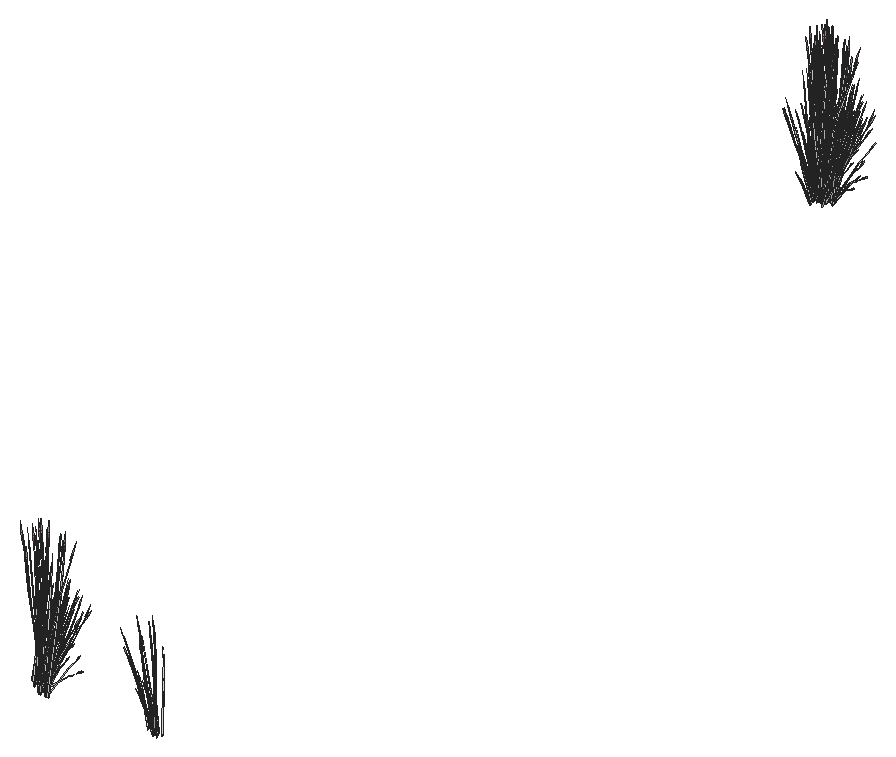
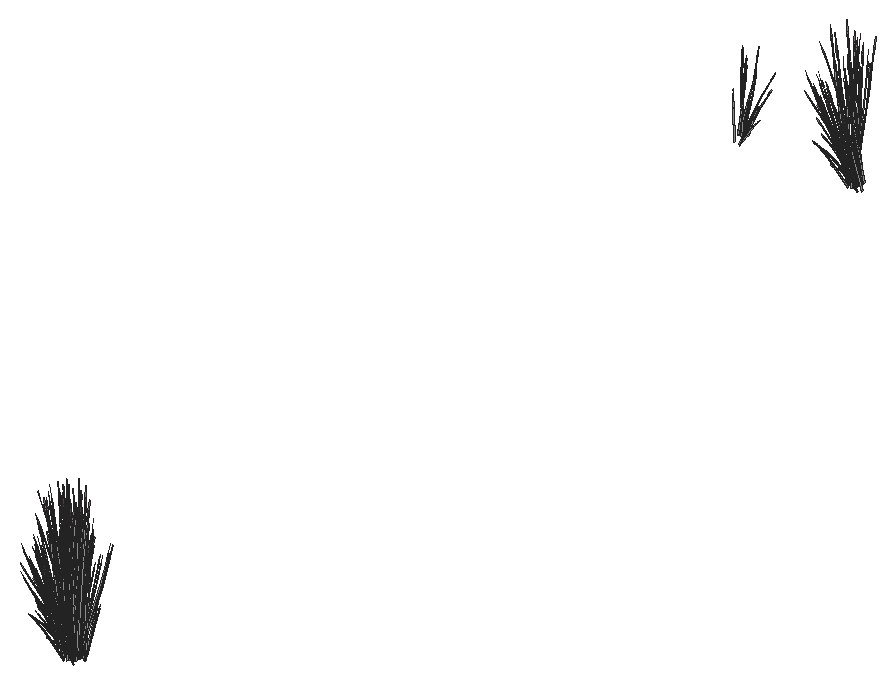
# SketchUp Ruby script. Lengths in inches.
U = 1.inch
M = Sketchup.active_model
def pt(a) = Geom::Point3d.new(a.map { |v| v * U })
def face(e, loops, mat)
  f = e.add_face(loops[0].map { |a| pt(a) })
  loops[1..].each { |l| e.add_face(l.map { |a| pt(a) }).erase! }
  f.material = f.back_material = mat if mat
  f
end
# faces: each face lists its corners as indices into pts; further lists are holes
def faces(e, pts, list, mat = nil) = list.each { |f| face(e, (f[0].is_a?(Array) ? f : [f]).map { |l| l.map { |i| pts[i] } }, mat) }
# xy, xz, yz: faces in a plane at the given z, y or x. An outline is a flat list of corners, or four numbers for a rectangle; further outlines are holes
def ring(l) = l.size == 4 ? [[l[0], l[1]], [l[2], l[1]], [l[2], l[3]], [l[0], l[3]]] : l.each_slice(2).to_a
def flat(e, list, mat, &to3) = list.each { |f| face(e, (f[0].is_a?(Array) ? f : [f]).map { |l| ring(l).map { |u, v| to3.(u, v) } }, mat) }
def xy(e, z, list, mat = nil) = flat(e, list, mat) { |x, y| [x, y, z] }
def xz(e, y, list, mat = nil) = flat(e, list, mat) { |x, z| [x, y, z] }
def yz(e, x, list, mat = nil) = flat(e, list, mat) { |y, z| [x, y, z] }
def lines(e, pts, list) = list.each { |a, b| e.add_line(pt(pts[a]), pt(pts[b])) }
# prism: a flat outline (further loops are holes) pulled along v
def prism(e, loops, v, mat = nil)
  f = face(e, loops, mat); d = Geom::Vector3d.new(v.map { |x| x * U })
  f.pushpull(f.normal.samedirection?(d) ? d.length : -d.length)
end
def box(e, o, s, mat = nil) = prism(e, [[o, [o[0] + s[0], o[1], o[2]], [o[0] + s[0], o[1] + s[1], o[2]], [o[0], o[1] + s[1], o[2]]]], [0, 0, s[2]], mat)
def at(x, y, z, deg = 0) = Geom::Transformation.translation(pt([x, y, z])) * Geom::Transformation.rotation(ORIGIN, Z_AXIS, deg.degrees)
def axes(o, x, y, z) = Geom::Transformation.new([*x, 0, *y, 0, *z, 0, *pt(o).to_a, 1])
def part(name) = M.definitions.add(name)
# library, detail: a bought-in or finely detailed component or shape, given as its bounding box
def library(name, o, s) = part(name).tap { |d| box(d.entities, o, s) }
def detail(e, o, s) = box(e.add_group.entities, o, s)
def put(e, d, t, mat = nil) = e.add_instance(d, t).tap { |i| i.material = mat if mat }
def group(e, t, mat = nil) = e.add_group.tap { |g| g.transformation = t; g.material = mat if mat }.entities
root = M.entities
M.materials.add("LightPink_Translucent").color = [144, 107, 117]
M.materials["LightPink_Translucent"].alpha = 0.75
c1 = part("blade")
p = [[2.15,0.21,22],[0,0.17,0],[0.09,0.45,0],[2.18,0.31,22],[2.29,0.31,22],[0.38,0.45,0],
  [2.48,0.24,33],[2.49,0.24,33],[2.48,0.22,33]]
faces(c1.entities,p,[[0,1,2,3],[4,5,2,3],[6,3,4,7],[8,0,3,6]])
c2 = part("seeds")
p = [[0.3,-0.1,1.38],[-0.01,-0.03,1.59],[-0.01,-0.03,0.03],[0.14,-0.07,-0.07],[0.29,-0.03,3],[0.15,0.01,3.11]]
faces(c2.entities,p,[[0,1,2,3],[1,0,4,5]],"LightPink_Translucent")
c3 = part("blade with seeds")
put(c3.entities,c1,at(0,0,0))
put(c3.entities,c2,axes([2.4,0.25,30.99],[1.5799,-0.05474,1.17369],[-0.12525,1.92788,0.29478],[-0.07173,-0.02425,1.56792]))
put(root,c3,axes([698.92,479.98,4.52],[-0.44971,0.15222,-0.0608],[-0.221,-0.27017,-0.33747],[-0.05933,-0.11385,0.51278]))
put(root,c3,axes([698.54,480,4.34],[-0.45175,-0.08196,-0.25549],[0.15485,-0.28101,-0.1979],[-0.04142,-0.11314,0.48886]))
put(root,c3,axes([697.7,482.08,3.9375],[-0.01125,-0.12549,0.85688],[0.48751,0.08325,0.06928],[-0.03015,0.17883,0.36631]))
put(root,c3,axes([696.8,481.01,3.01],[0.32079,-0.20399,-0.15489],[0.32079,0.20399,0.15489],[0,-0.06571,0.69487]))
put(root,c3,axes([699.8,281.16,1.01],[-0.4301,0.16348,-0.24825],[-0.25708,-0.29314,0],[-0.09796,0.03723,0.78752]))
put(root,c3,axes([698.24,479.69,3.0625],[-0.31757,0.18757,-0.01946],[-0.29098,-0.20543,-0.08825],[-0.02049,-0.05821,0.29107]))
put(root,c3,axes([699.83,281.07,1.1],[-0.28374,-0.32877,-0.02571],[0.4807,-0.18271,0.25804],[-0.11845,0.0313,0.81815]))
put(root,c3,axes([698.12,481.54,3.18],[0.58084,0.06889,0.22877],[-0.11821,0.38906,0.08977],[-0.08488,-0.03757,0.79428]))
put(root,c3,axes([698.01,280.92,2.5],[0.32898,0.21969,-0.2836],[-0.34753,0.1924,-0.21967],[-0.05006,0.11162,0.54264]))
put(root,c3,axes([699.7,281.03,1.01],[-0.42874,-0.0809,-0.15489],[0.10795,-0.28489,0.15489],[-0.08643,0.03285,0.69487]))
put(root,c3,axes([697.97,481.47,3.36],[-0.22297,0.29461,0.2237],[-0.4633,-0.14179,-0.10766],[0,-0.06791,0.71822]))
put(root,c3,axes([698.7,480.05,4.49],[-0.21934,-0.26585,-0.35523],[0.45151,-0.14816,0.04287],[-0.05129,-0.12845,0.5025]))
put(root,c3,axes([697.86,280.76,2.53],[0.31095,-0.17214,0.17707],[0.29435,0.19656,-0.2286],[-0.04479,0.09987,0.4374]))
put(root,c3,axes([699.95,279.81,1.42],[-0.01255,-0.30784,0.70636],[0.56816,0.0798,0.29908],[-0.13438,0.16845,0.66675]))
put(root,c3,axes([697.8,482.16,3.24],[0.49383,-0.08678,0.08821],[0.12194,0.32295,0.17543],[-0.04404,-0.04705,0.80203]))
put(root,c3,axes([697.66,280.81,2.7],[0.50507,0.0162,-0.06749],[-0.01381,0.30672,-0.3746],[-0.03508,0.11813,0.56919]))
put(root,c3,axes([697.65,281.25,1.41],[0.41748,-0.0579,0.03254],[0.09598,0.23326,-0.43152],[-0.02647,0.11808,0.3868]))
put(root,c3,axes([699.625,280.2,1.33],[0.05355,0.37308,-0.14548],[-0.55775,0.02256,-0.25001],[-0.09822,0.04969,0.79854]))
put(root,c3,axes([698.44,482.21,3.1],[-0.4633,-0.14679,0],[0.22297,-0.30501,0],[0,0,0.81353]))
put(root,c3,axes([698.79,480.09,4.53],[-0.13855,0.25143,0.17707],[-0.4042,-0.07334,-0.2286],[-0.03706,-0.10123,0.4374]))
put(root,c3,axes([699.51,482.58,3.1875],[0.28732,0.32763,0],[-0.4807,0.18271,-0.25804],[-0.10948,0.04161,0.81856]))
put(root,c3,axes([698.38,280.61,1.9375],[-0.01125,-0.12549,0.85688],[0.48751,0.08325,0.06928],[-0.03015,0.17883,0.36631]))
put(root,c3,axes([698.05,482.72,4.53],[-0.45283,-0.08548,0.26641],[0.15485,-0.28101,0.21967],[0.02721,0.11051,0.55128]))
put(root,c3,axes([697.93,482.74,4.37],[-0.33863,0.11112,0.03215],[-0.16575,-0.20263,0.2531],[0.0327,0.08932,0.38595]))
put(root,c3,axes([699.27,482.18,3.24],[0.13276,-0.32494,0.08821],[0.4858,0.09195,0.17543],[-0.08392,0.00158,0.80203]))
put(root,c3,axes([699.05,481.75,3.31],[0.33952,0.19644,0.0724],[-0.2832,0.22163,-0.20674],[-0.07883,0.02996,0.63372]))
put(root,c3,axes([698.93,481.51,3.15],[-0.42746,-0.28142,-0.03066],[0.42772,-0.28159,0],[-0.01493,-0.00983,0.87786]))
put(root,c3,axes([699.04,481.6,3.36],[0.49904,-0.02018,0.2237],[0.04513,0.33504,-0.10766],[-0.08934,0.03396,0.71822]))
put(root,c3,axes([699.16,482.375,3.17],[0.57533,0.10627,0.15378],[-0.14394,0.37986,-0.18246],[-0.09522,0.04754,0.82443]))
put(root,c3,axes([698.32,479.46,2.75],[-0.07708,0.01178,0.88171],[-0.42627,-0.1326,-0.1347],[0.00715,-0.1106,0.15018]))
put(root,c3,axes([699.41,482.35,3.24],[0.4301,-0.16348,0.24825],[0.25708,0.29314,0],[-0.09796,0.03723,0.78752]))
put(root,c3,axes([698.74,479.82,4.26],[0.13855,-0.25143,-0.17707],[0.4042,0.07334,0.2286],[-0.03706,-0.10123,0.4374]))
put(root,c3,axes([698.07,481.18,3.18],[0.1998,0.3656,0.22877],[-0.5709,0.12713,0.08977],[0.00698,-0.06718,0.79428]))
put(root,c3,axes([697.98,481.14,3.11],[0.22297,-0.29461,-0.2237],[0.4633,0.14179,0.10766],[0,-0.06791,0.71822]))
put(root,c3,axes([698.55,482.09,3.1],[-0.14994,-0.28188,0],[0.42817,-0.09871,0],[0,0,0.77185]))
put(root,c3,axes([698,482.68,2.75],[0.07437,-0.01779,0.88171],[0.44738,0.09793,-0.1347],[0.01308,0.11037,0.15018]))
put(root,c3,axes([698.1,482.78,4.26],[-0.13855,0.25143,-0.17707],[-0.4042,-0.07334,0.2286],[0.03706,0.10123,0.4374]))
put(root,c3,axes([700.19,281.11,1.1875],[0.28732,0.32763,0],[-0.4807,0.18271,-0.25804],[-0.10948,0.04161,0.81856]))
put(root,c3,axes([698.73,281.25,2.53],[-0.45283,-0.08548,0.26641],[0.15485,-0.28101,0.21967],[0.02721,0.11051,0.55128]))
put(root,c3,axes([698.61,281.27,2.37],[-0.33863,0.11112,0.03215],[-0.16575,-0.20263,0.2531],[0.0327,0.08932,0.38595]))
put(root,c3,axes([699.73,280.27,1.31],[0.33952,0.19644,0.0724],[-0.2832,0.22163,-0.20674],[-0.07883,0.02996,0.63372]))
put(root,c3,axes([699.15,481.53,3.11],[-0.22297,0.29461,-0.2237],[-0.4633,-0.14179,0.10766],[0,0.06791,0.71822]))
put(root,c3,axes([698.91,479.86,4.37],[0.33863,-0.11112,0.03215],[0.16575,0.20263,0.2531],[-0.0327,-0.08932,0.38595]))
put(root,c3,axes([697.8125,483.23,4.36],[0.05825,0.05265,0.87472],[0.47011,0.02068,-0.13834],[0.04727,0.11612,0.07015]))
put(root,c3,axes([700.03,481.35,3.24],[-0.36107,-0.23816,0.08821],[0.36387,-0.231,0.17543],[-0.03988,0.04864,0.80203]))
put(root,c3,axes([698.79,481.21,3.1],[0,-0.37831,0],[0.57465,0,0],[0,0,0.89728]))
put(root,c3,axes([699.84,280.9,1.17],[0.57533,0.10627,0.15378],[-0.14394,0.37986,-0.18246],[-0.09522,0.04754,0.82443]))
put(root,c3,axes([698.79,479.88,4.37],[0.45283,0.08548,0.24001],[-0.15485,0.28101,0.1979],[-0.02721,-0.11051,0.49665]))
put(root,c3,axes([698.25,481.28,3.22],[0.5178,0.15847,0.12032],[-0.2492,0.32927,0.25001],[0,-0.0759,0.80271]))
put(root,c3,axes([699.07,481.36,3.15],[0,0.37813,-0.02818],[-0.57465,0,0],[0,0.01188,0.89684]))
put(root,c3,axes([698.08,481.0625,3.36],[-0.49904,0.02018,0.2237],[-0.04513,-0.33504,-0.10766],[0.08934,-0.03396,0.71822]))
put(root,c3,axes([700.09,280.88,1.24],[0.4301,-0.16348,0.24825],[0.25708,0.29314,0],[-0.09796,0.03723,0.78752]))
put(root,c3,axes([698.06,482.51,4.53],[0.13855,-0.25143,0.17707],[0.4042,0.07334,-0.2286],[0.03706,0.10123,0.4374]))
put(root,c3,axes([697.85,480.49,3.24],[-0.13276,0.32494,0.08821],[-0.4858,-0.09195,0.17543],[0.08392,-0.00158,0.80203]))
put(root,c3,axes([698.8,482.1,3.15],[0.1998,0.37562,-0.03006],[-0.5709,0.13162,0],[0.00698,0.01312,0.86086]))
put(root,c3,axes([698.68,281.21,0.75],[0.07437,-0.01779,0.88171],[0.44738,0.09793,-0.1347],[0.01308,0.11037,0.15018]))
put(root,c3,axes([698.78,281.31,2.26],[-0.13855,0.25143,-0.17707],[-0.4042,-0.07334,0.2286],[0.03706,0.10123,0.4374]))
put(root,c3,axes([697.61,480.08,3.1875],[-0.28732,-0.32763,0],[0.4807,-0.18271,-0.25804],[0.10948,-0.04161,0.81856]))
put(root,c3,axes([698.14,482.55,4.49],[0.21934,0.26585,-0.35523],[-0.45151,0.14816,0.04287],[0.05129,0.12845,0.5025]))
put(root,c3,axes([700.45,481.6,3.1],[-0.57436,-0.00261,-0.02488],[0,-0.36542,0.24971],[-0.01805,0.08319,0.79176]))
put(root,c3,axes([699.32,480.5,3.24],[-0.49383,0.08678,0.08821],[-0.12194,-0.32295,0.17543],[0.04404,0.04705,0.80203]))
put(root,c3,axes([699.83,280.06,1.11],[-0.22297,0.29461,-0.2237],[-0.4633,-0.14179,0.10766],[0,0.06791,0.71822]))
put(root,c3,axes([698.82,479.29,3.38],[0.05895,0.19066,0.5743],[-0.32704,-0.1056,0.42196],[0.03519,-0.09762,0.12649]))
put(root,c3,axes([698.6,483.41,4.82],[0.31757,-0.18757,-0.03244],[0.29098,0.20543,-0.14708],[0.02049,0.05821,0.48512]))
put(root,c3,axes([698.49,281.75,2.36],[0.05825,0.05265,0.87472],[0.47011,0.02068,-0.13834],[0.04727,0.11612,0.07015]))
put(root,c3,axes([698.51,480.97,3.18],[-0.38104,0.29672,0.22877],[-0.45269,-0.26192,0.08977],[0.09186,-0.02961,0.79428]))
put(root,c3,axes([699.16,481.44,3.11],[0.32079,0.21119,0],[-0.32079,0.21119,0],[0,0,0.84633]))
put(root,c3,axes([699.16,481.19,3.36],[0.22297,-0.29461,0.2237],[0.4633,0.14179,-0.10766],[0,0.06791,0.71822]))
put(root,c3,axes([698.97,482.22,3.1],[0.4633,0.14679,0],[-0.22297,0.30501,0],[0,0,0.87477]))
put(root,c3,axes([698.31,482.61,4.34],[0.45175,0.08196,-0.25549],[-0.15485,0.28101,-0.1979],[0.04142,0.11314,0.48886]))
put(root,c3,axes([698.73,281.04,2.53],[0.13855,-0.25143,0.17707],[0.4042,0.07334,-0.2286],[0.03706,0.10123,0.4374]))
put(root,c3,axes([697.92,482.62,4.52],[0.44971,-0.15222,-0.0608],[0.221,0.27017,-0.33747],[0.05933,0.11385,0.51278]))
put(root,c3,axes([699.01,481.125,3.19],[-0.58084,-0.06889,0.24599],[0.11821,-0.38906,0.09653],[0.08488,0.03757,0.85407]))
put(root,c3,axes([700.22,479.6,4.35],[-0.04667,0.02497,0.88692],[-0.45726,-0.08426,-0.08381],[-0.01655,-0.10898,0.15695]))
put(root,c3,axes([699.86,480.32,4.52],[-0.50507,-0.0162,-0.0608],[0.01381,-0.30672,-0.33747],[0.03508,-0.11813,0.51278]))
put(root,c3,axes([699.48,280.62,1.15],[0.1998,0.37562,-0.03006],[-0.5709,0.13162,0],[0.00698,0.01312,0.86086]))
put(root,c3,axes([700.33,481.66,3.01],[-0.32079,0.20399,-0.15489],[-0.32079,-0.20399,0.15489],[0,0.06571,0.69487]))
put(root,c3,axes([699.41,481.62,3.05],[0.16851,0.29936,-0.34606],[-0.4854,0.10781,-0.09083],[0.01863,0.10137,0.76386]))
put(root,c3,axes([699.18,481.3,3.1],[0.51416,0,0],[0,0.33849,0],[0,0,0.89203]))
put(root,c3,axes([699.66,480.37,4.53],[-0.31095,0.17214,0.17707],[-0.29435,-0.19656,-0.2286],[0.04479,-0.09987,0.4374]))
put(root,c3,axes([698.82,281.08,2.49],[0.21934,0.26585,-0.35523],[-0.45151,0.14816,0.04287],[0.05129,0.12845,0.5025]))
put(root,c3,axes([701.13,280.13,1.1],[-0.57436,-0.00261,-0.02488],[0,-0.36542,0.24971],[-0.01805,0.08319,0.79176]))
put(root,c3,axes([698.68,480.92,3.36],[-0.27607,-0.27443,0.2237],[0.41817,-0.19325,-0.10766],[0.08934,0.03396,0.71822]))
put(root,c3,axes([698.18,480.99,3.33],[-0.05355,-0.37308,-0.14548],[0.55775,-0.02256,-0.25001],[0.09822,-0.04969,0.79854]))
put(root,c3,axes([699.35,481.26,3.31],[0.42817,-0.09535,0.0724],[0.14994,0.27228,-0.20674],[0,0.05992,0.63372]))
put(root,c3,axes([699.51,480.21,4.34],[-0.32898,-0.21969,-0.25549],[0.34753,-0.1924,-0.1979],[0.05006,-0.11162,0.48886]))
put(root,c3,axes([699.28,281.9375,2.82],[0.31757,-0.18757,-0.03244],[0.29098,0.20543,-0.14708],[0.02049,0.05821,0.48512]))
put(root,c3,axes([699.21,481.28,3.33],[0.51755,0.15601,-0.14548],[-0.2492,0.32927,-0.25001],[0.01626,0.08084,0.79854]))
put(root,c3,axes([698.1,480.16,3.01],[0.42874,0.0809,-0.15489],[-0.10795,0.28489,0.15489],[0.08643,-0.03285,0.69487]))
put(root,c3,axes([699.3,479.82,3.3],[-0.13063,0.06618,0.71501],[-0.39122,-0.11583,-0.15377],[0.07252,-0.14406,0.3057]))
put(root,c3,axes([698.98,281.13,2.34],[0.45175,0.08196,-0.25549],[-0.15485,0.28101,-0.1979],[0.04142,0.11314,0.48886]))
put(root,c3,axes([698.6,281.15,2.52],[0.44971,-0.15222,-0.0608],[0.221,0.27017,-0.33747],[0.05933,0.11385,0.51278]))
put(root,c3,axes([700.33,481.36,3.24],[0,-0.32696,0.24825],[0.51416,0,0],[0,0.07447,0.78752]))
put(root,c3,axes([700.55,481.66,3.01],[0,0.32696,-0.24825],[-0.51416,0,0],[0,0.07447,0.78752]))
put(root,c3,axes([699.18,482.65,4.37],[-0.45708,0.07503,0.24001],[-0.07933,-0.29434,0.1979],[0.1075,0.08675,0.49665]))
put(root,c3,axes([698,480.03,3.01],[0.4301,-0.16348,-0.24825],[0.25708,0.29314,0],[0.09796,-0.03723,0.78752]))
put(root,c3,axes([699.09,482.71,4.37],[-0.20887,0.2077,0.03215],[-0.29744,-0.12092,0.2531],[0.09616,0.06659,0.38595]))
put(root,c3,axes([701.01,280.18,1.01],[-0.32079,0.20399,-0.15489],[-0.32079,-0.20399,0.15489],[0,0.06571,0.69487]))
put(root,c3,axes([698.5625,482.03,3.9375],[-0.10505,-0.10498,0.85688],[0.48542,-0.08838,0.06928],[0.10971,0.1648,0.36631]))
put(root,c3,axes([698.87,480.85,3.31],[0.08866,-0.29179,0.0724],[0.43315,0.05065,-0.20674],[0.07883,0.02996,0.63372]))
put(root,c3,axes([700.09,280.14,1.05],[0.16851,0.29936,-0.34606],[-0.4854,0.10781,-0.09083],[0.01863,0.10137,0.76386]))
put(root,c3,axes([699.48,480.34,3.24],[-0.4301,-0.16348,0.24825],[0.25708,-0.29314,0],[0.09796,0.03723,0.78752]))
put(root,c3,axes([699.62,480.31,4.49],[0.01196,-0.30243,-0.35523],[0.50354,0.02031,0.04287],[0.05314,-0.12813,0.5025]))
put(root,c3,axes([699.11,482.05,3.09],[0.48247,-0.11094,-0.09599],[0.16954,0.31956,0.00004],[0.05326,-0.01226,0.86949]))
put(root,c3,axes([699.88,279.8125,1.33],[0.51755,0.15601,-0.14548],[-0.2492,0.32927,-0.25001],[0.01626,0.08084,0.79854]))
put(root,c3,axes([699.03,482.47,4.53],[-0.07098,-0.26335,0.17707],[0.40574,-0.06954,-0.2286],[0.10898,0.07547,0.4374]))
put(root,c3,axes([699.12,481.1,3.11],[0.27607,0.27443,-0.2237],[-0.41817,0.19325,0.10766],[0.08934,0.03396,0.71822]))
put(root,c3,axes([701.23,280.1875,1.01],[0,0.32696,-0.24825],[-0.51416,0,0],[0,0.07447,0.78752]))
put(root,c3,axes([699.86,281.18,2.37],[-0.45708,0.07503,0.24001],[-0.07933,-0.29434,0.1979],[0.1075,0.08675,0.49665]))
put(root,c3,axes([699.3,480.96,4.24],[-0.39711,-0.16988,0.69141],[0.41931,-0.2645,0.29833],[0.12812,0.1594,0.66832]))
put(root,c3,axes([699.82,480.13,4.26],[0.31095,-0.17214,-0.17707],[0.29435,0.19656,0.2286],[0.04479,-0.09987,0.4374]))
put(root,c3,axes([699.77,281.24,2.37],[-0.20887,0.2077,0.03215],[-0.29744,-0.12092,0.2531],[0.09616,0.06659,0.38595]))
put(root,c3,axes([699.24,280.55,1.9375],[-0.10505,-0.10498,0.85688],[0.48542,-0.08838,0.06928],[0.10971,0.1648,0.36631]))
put(root,c3,axes([698.63,482.84,4.35],[0.00136,-0.03958,0.88692],[0.39383,-0.17464,-0.08381],[0.1368,0.06234,0.15695]))
put(root,c3,axes([699.94,480.22,4.37],[0.37765,0.01523,0.03215],[-0.01035,0.23004,0.2531],[0.03952,-0.08812,0.38595]))
put(root,c3,axes([699.9,482.34,3.38],[-0.25875,-0.09401,0.5743],[0.33411,-0.09552,0.42196],[0.09012,0.08091,0.12649]))
put(root,c3,axes([698.98,482.24,3.3],[0.00811,-0.10838,0.71501],[0.38755,-0.12106,-0.15377],[0.11964,0.12972,0.3057]))
put(root,c3,axes([700.32,479.84,4.36],[-0.00444,-0.06507,0.87472],[-0.37468,-0.18807,-0.13834],[0.05793,-0.114,0.07015]))
put(root,c3,axes([698.51,480.7,3.03],[0.30954,-0.24575,-0.31177],[0.38452,0.22284,-0.08182],[0.12404,-0.0613,0.68817]))
put(root,c3,axes([699.82,480.19,4.37],[0.32725,0.22308,0.24001],[-0.34753,0.1924,0.1979],[0.06036,-0.10466,0.49665]))
put(root,c3,axes([699.87,480.49,3.01],[0.10795,0.28489,-0.15489],[-0.42874,0.0809,0.15489],[0.08643,0.03285,0.69487]))
put(root,c3,axes([700.68,481.41,3.1875],[0.57465,0,0],[0,0.36542,-0.25804],[0,0.08323,0.81856]))
put(root,c3,axes([698.82,480.94,3.33],[0.46399,-0.21707,-0.14548],[0.30855,0.30672,-0.25001],[0.11448,0.03115,0.79854]))
put(root,c3,axes([699.7,281,2.53],[-0.07098,-0.26335,0.17707],[0.40574,-0.06954,-0.2286],[0.10898,0.07547,0.4374]))
put(root,c3,axes([699.9375,482.77,3.33],[-0.2947,-0.01025,0.5253],[0.19462,-0.21779,0.29003],[0.11642,0.07737,0.41205]))
put(root,c3,axes([700.2,480.9,4.53],[-0.40003,0.04673,0.17707],[-0.10563,-0.26712,-0.2286],[0.11464,-0.07175,0.4374]))
put(root,c3,axes([699.05,480.16,3.9375],[-0.08557,0.11238,0.85688],[-0.35897,-0.23257,0.06928],[0.16194,-0.14495,0.36631]))
put(root,c3,axes([699.98,279.48,2.24],[-0.39711,-0.16988,0.69141],[0.41931,-0.2645,0.29833],[0.12812,0.1594,0.66832]))
put(root,c3,axes([699.31,281.37,2.35],[0.00136,-0.03958,0.88692],[0.39383,-0.17464,-0.08381],[0.1368,0.06234,0.15695]))
put(root,c3,axes([700.58,280.87,1.38],[-0.25875,-0.09401,0.5743],[0.33411,-0.09552,0.42196],[0.09012,0.08091,0.12649]))
put(root,c3,axes([699.65,280.77,1.3],[0.00811,-0.10838,0.71501],[0.38755,-0.12106,-0.15377],[0.11964,0.12972,0.3057]))
put(root,c3,axes([698.99,482.61,4.52],[0.27385,-0.27986,-0.0608],[0.39658,0.16123,-0.33747],[0.13785,0.07907,0.51278]))
put(root,c3,axes([697.65,480.75,2.8],[-0.45234,0.1309,0.64464],[-0.14398,-0.37559,0.25048],[0.27777,0.00625,0.73321]))
put(root,c3,axes([700.41,480.93,4.52],[-0.4251,-0.18028,-0.0608],[0.24491,-0.26108,-0.33747],[0.1201,-0.09075,0.51278]))
put(root,c3,axes([701.36,279.94,1.1875],[0.57465,0,0],[0,0.36542,-0.25804],[0,0.08323,0.81856]))
put(root,c3,axes([699.3125,482.47,4.34],[0.45348,-0.07772,-0.25549],[0.07933,0.29434,-0.1979],[0.1218,0.08435,0.48886]))
put(root,c3,axes([699.73,480.17,3.1875],[0.28732,-0.32763,0],[0.4807,0.18271,-0.25804],[0.10948,0.04161,0.81856]))
put(root,c3,axes([700.21,480.02,2.75],[-0.06878,-0.02576,0.88171],[-0.17668,-0.28776,-0.1347],[0.11919,-0.07809,0.15018]))
put(root,c3,axes([699.83,482.12,4.53],[-0.26148,-0.20471,0.17707],[0.29857,-0.19378,-0.2286],[0.1517,0.02948,0.4374]))
put(root,c3,axes([699.99,480.36,3.01],[0.4301,0.16348,-0.24825],[-0.25708,0.29314,0],[0.09796,0.03723,0.78752]))
put(root,c3,axes([700.62,281.3,1.33],[-0.2947,-0.01025,0.5253],[0.19462,-0.21779,0.29003],[0.11642,0.07737,0.41205]))
put(root,c3,axes([700.07,482.3,4.37],[-0.02314,0.24862,0.03215],[-0.34943,-0.00682,0.2531],[0.13385,0.02602,0.38595]))
put(root,c3,axes([699.97,482.69,2.75],[0.03348,-0.0472,0.88171],[0.42153,-0.13902,-0.1347],[0.12779,0.07195,0.15018]))
put(root,c3,axes([700.1,482.22,4.37],[-0.33886,0.21544,0.24001],[-0.29224,-0.22879,0.1979],[0.15898,0.03974,0.49665]))
put(root,c3,axes([700.2,480.72,4.34],[-0.11806,-0.29854,-0.25549],[0.44709,-0.05222,-0.1979],[0.12812,-0.08019,0.48886]))
put(root,c3,axes([700.98,482.26,3.96],[-0.08796,-0.27485,-0.01746],[0.41573,-0.06319,-0.07916],[0.08682,0.01742,0.26109]))
put(root,c3,axes([700.26,481.54,4.53],[-0.38192,-0.09121,0.17707],[0.11139,-0.2661,-0.2286],[0.15377,-0.0244,0.4374]))
put(root,c3,axes([699.36,480.99,3.03],[0.47805,0.0536,-0.31177],[-0.10088,0.33065,-0.08182],[0.14266,0.04007,0.68817]))
put(root,c3,axes([699.67,281.14,2.52],[0.27385,-0.27986,-0.0608],[0.39658,0.16123,-0.33747],[0.13785,0.07907,0.51278]))
put(root,c3,axes([701.4,481.19,3.13],[-0.28491,-0.20907,-0.03244],[0.31204,-0.19157,-0.14708],[0.08842,-0.01349,0.48512]))
put(root,c3,axes([700.75,480.12,3.38],[-0.15307,0.16644,0.5743],[-0.13157,-0.22361,0.42196],[0.12643,-0.05603,0.12649]))
put(root,c3,axes([700.5625,480.86,4.37],[0.31549,0.13751,0.03215],[-0.18368,0.19581,0.2531],[0.10115,-0.06331,0.38595]))
put(root,c3,axes([699.99,281,2.34],[0.45348,-0.07772,-0.25549],[0.07933,0.29434,-0.1979],[0.1218,0.08435,0.48886]))
put(root,c3,axes([700.48,480.8,4.37],[0.11397,0.30091,0.24001],[-0.44709,0.05222,0.1979],[0.13177,-0.07077,0.49665]))
put(root,c3,axes([700.75,280.83,2.37],[-0.02314,0.24862,0.03215],[-0.34943,-0.00682,0.2531],[0.13385,0.02602,0.38595]))
put(root,c3,axes([699.27,481.7,3.9375],[-0.1707,-0.05633,0.85688],[0.35326,-0.23632,0.06928],[0.22018,0.10661,0.36631]))
put(root,c3,axes([700.65,281.22,0.75],[0.03348,-0.0472,0.88171],[0.42153,-0.13902,-0.1347],[0.12779,0.07195,0.15018]))
put(root,c3,axes([700.78,280.75,2.37],[-0.33886,0.21544,0.24001],[-0.29224,-0.22879,0.1979],[0.15898,0.03974,0.49665]))
put(root,c3,axes([701.45,480.85,4.35],[-0.06002,-0.00248,0.88692],[-0.24926,-0.26607,-0.08381],[0.1001,-0.08748,0.15695]))
put(root,c3,axes([700.53,480.75,4.26],[0.40003,-0.04673,-0.17707],[0.10563,0.26712,0.2286],[0.11464,-0.07175,0.4374]))
put(root,c3,axes([700.21,480.84,4.49],[0.24005,-0.25798,-0.35523],[0.42065,0.18334,0.04287],[0.14333,-0.09347,0.5025]))
put(root,c3,axes([700.61,481.625,4.37],[0.16879,0.22293,0.03215],[-0.30779,0.10912,0.2531],[0.13568,-0.02153,0.38595]))
put(root,c3,axes([700.2,482.22,4.26],[0.26148,0.20471,-0.17707],[-0.29857,0.19378,0.2286],[0.1517,0.02948,0.4374]))
put(root,c3,axes([699.91,482.25,4.52],[0.02461,-0.33251,-0.0608],[0.4659,0.00909,-0.33747],[0.17944,0.0231,0.51278]))
put(root,c3,axes([700.43,481.63,4.52],[-0.23123,-0.29606,-0.0608],[0.41039,-0.14549,-0.33747],[0.17294,-0.03906,0.51278]))
put(root,c3,axes([700.58,481.55,4.37],[-0.12984,0.29812,0.24001],[-0.42685,-0.10194,0.1979],[0.16786,-0.01792,0.49665]))
put(root,c3,axes([700.3125,482.05,4.36],[0.09858,-0.00553,0.87472],[0.2704,-0.25401,-0.13834],[0.17535,0.03353,0.07015]))
put(root,c3,axes([699.94,280.23,1.9375],[-0.1707,-0.05633,0.85688],[0.35326,-0.23632,0.06928],[0.22018,0.10661,0.36631]))
put(root,c3,axes([700.4,481.38,4.34],[0.1245,-0.29741,-0.25549],[0.42685,0.10194,-0.1979],[0.17186,-0.02727,0.48886]))
put(root,c3,axes([701.48,481.57,3.38],[-0.28394,0.05398,0.5743],[0.13365,-0.22308,0.42196],[0.15063,0.01526,0.12649]))
put(root,c3,axes([700.56,480.6,3.3],[-0.16417,-0.00968,0.71501],[-0.16819,-0.25979,-0.15377],[0.20169,-0.07349,0.3057]))
put(root,c3,axes([700.88,280.75,2.26],[0.26148,0.20471,-0.17707],[-0.29857,0.19378,0.2286],[0.1517,0.02948,0.4374]))
put(root,c3,axes([700.67,481.51,4.26],[0.38192,0.09121,-0.17707],[-0.11139,0.2661,0.2286],[0.15377,-0.0244,0.4374]))
put(root,c3,axes([699.93,482.09,4.49],[0.45939,0.00787,-0.35523],[-0.03085,0.3315,0.04287],[0.19462,0.03498,0.5025]))
put(root,c3,axes([700.86,481.46,2.99],[-0.29599,0.03924,0.70792],[-0.04711,-0.31232,0.04052],[0.20731,-0.04727,0.40283]))
put(root,c3,axes([701.18,481.26,2.75],[-0.02402,-0.04964,0.88171],[0.16658,-0.29036,-0.1347],[0.16804,-0.00418,0.15018]))
put(root,c3,axes([701.34,482.51,4.35],[-0.04155,-0.02862,0.88692],[0.0909,-0.30682,-0.08381],[0.16368,-0.0196,0.15695]))
put(root,c3,axes([699.625,481.18,3.9375],[-0.19062,0.00741,0.85688],[0.12645,-0.32094,0.06928],[0.27165,0.01985,0.36631]))
put(root,c3,axes([700.99,280.57,2.36],[0.09858,-0.00553,0.87472],[0.2704,-0.25401,-0.13834],[0.17535,0.03353,0.07015]))
put(root,c3,axes([700.32,481.49,4.49],[0.40382,-0.1444,-0.35523],[0.22505,0.29724,0.04287],[0.19512,-0.03377,0.5025]))
put(root,c3,axes([701.68,481.17,4.36],[0.06377,-0.0498,0.87472],[-0.08162,-0.30549,-0.13834],[0.16001,-0.05792,0.07015]))
put(root,c3,axes([700.61,280.61,2.49],[0.45939,0.00787,-0.35523],[-0.03085,0.3315,0.04287],[0.19462,0.03498,0.5025]))
put(root,c3,axes([700.94,481.93,3.3],[-0.11068,-0.08041,0.71501],[0.144,-0.26601,-0.15377],[0.22393,0.03604,0.3057]))
put(root,c3,axes([723.21,279.86,1.9375],[0.15946,-0.06916,0.85688],[0.13424,0.31957,0.06928],[-0.25033,0.07223,0.36631]))
put(root,c3,axes([722.71,280.4,1.3],[0.15971,0.02684,0.71501],[0.10294,0.27415,-0.15377],[-0.21694,0.05132,0.3057]))
put(root,c3,axes([721.89,280.06,2.35],[0.05865,0.00877,0.88692],[0.18143,0.28888,-0.08381],[-0.12006,0.07582,0.15695]))
put(root,c3,axes([722.38,280.98,1.38],[0.19152,-0.14818,0.5743],[0.07557,0.23459,0.42196],[-0.13841,0.042,0.12649]))
put(root,c3,axes([723.79,280.07,1.9375],[0.11478,-0.10046,0.85688],[0.28982,0.27117,0.06928],[-0.19878,0.12349,0.36631]))
put(root,c3,axes([723.1,280.33,2.26],[-0.40003,0.04673,-0.17707],[-0.10563,-0.26712,0.2286],[-0.11464,0.07175,0.4374]))
put(root,c3,axes([722.88,281.13,0.75],[0.06164,0.03267,0.88171],[0.10452,0.30266,-0.1347],[-0.13662,0.06454,0.15018]))
put(root,c3,axes([723.15,280.28,2.37],[-0.11397,-0.30091,0.24001],[0.44709,-0.05222,0.1979],[-0.13177,0.07077,0.49665]))
put(root,c3,axes([723.07,280.22,2.37],[-0.31549,-0.13751,0.03215],[0.18368,-0.19581,0.2531],[-0.10115,0.06331,0.38595]))
put(root,c3,axes([723.71,280.32,1.9375],[0.08557,-0.11238,0.85688],[0.35897,0.23257,0.06928],[-0.16194,0.14495,0.36631]))
put(root,c3,axes([723.43,280.37,2.34],[0.11806,0.29854,-0.25549],[-0.44709,0.05222,-0.1979],[-0.12812,0.08019,0.48886]))
put(root,c3,axes([722.73,280.9,2.36],[-0.01142,0.0647,0.87472],[0.32418,0.22509,-0.13834],[-0.08487,0.10644,0.07015]))
put(root,c3,axes([723.22,280.15,2.52],[0.4251,0.18028,-0.0608],[-0.24491,0.26108,-0.33747],[-0.1201,0.09075,0.51278]))
put(root,c3,axes([722.52,280.93,2.82],[0.40553,0.08728,-0.03244],[-0.12475,0.26862,-0.14708],[-0.06633,0.04078,0.48512]))
put(root,c3,axes([723.43,280.18,2.53],[0.40003,-0.04673,0.17707],[0.10563,0.26712,-0.2286],[-0.11464,0.07175,0.4374]))
put(root,c3,axes([723.66,281.45,1.3],[0.14502,-0.05158,0.71501],[0.35805,0.15552,-0.15377],[-0.10657,0.13457,0.3057]))
